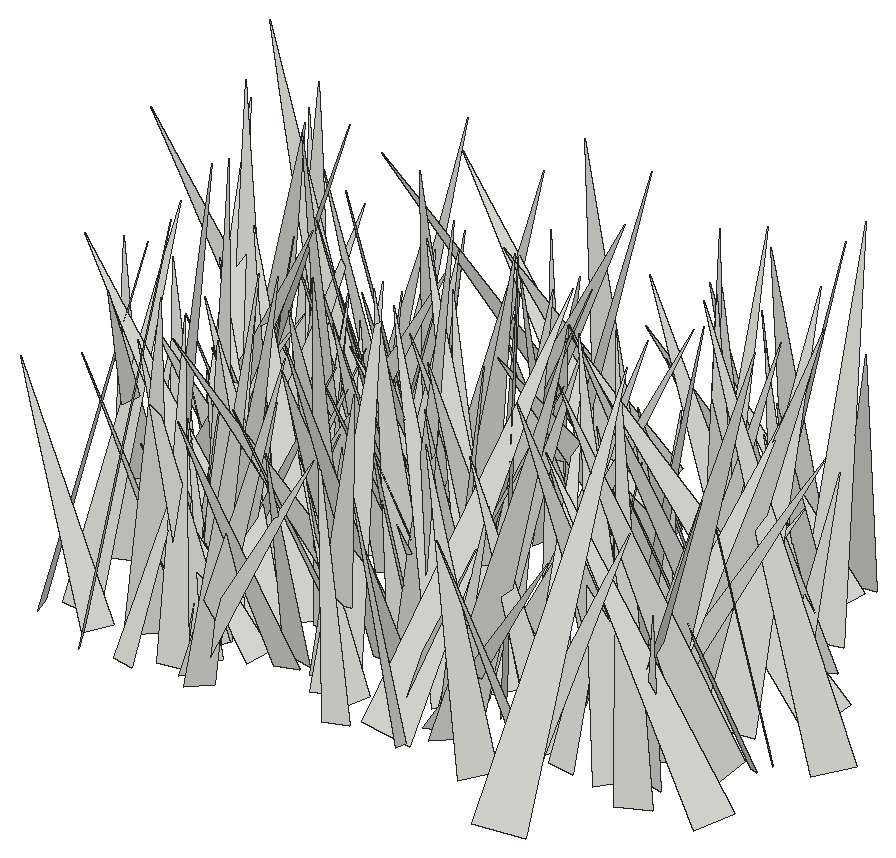
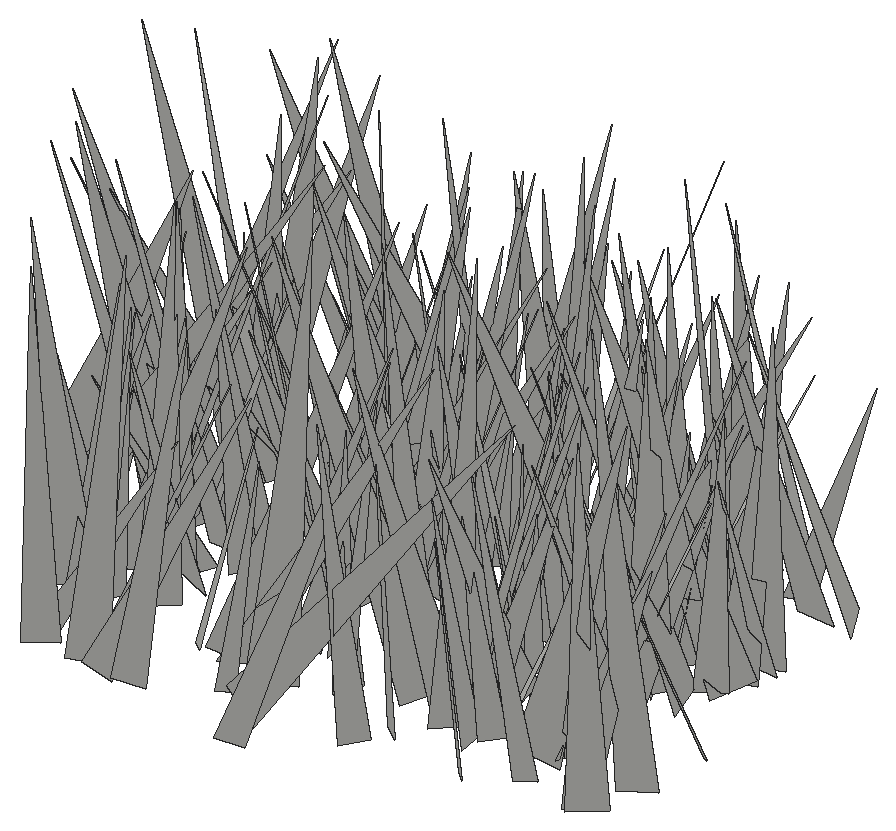
# SketchUp Ruby script. Lengths in inches.
U = 1.inch
M = Sketchup.active_model
def pt(a) = Geom::Point3d.new(a.map { |v| v * U })
def face(e, loops, mat)
  f = e.add_face(loops[0].map { |a| pt(a) })
  loops[1..].each { |l| e.add_face(l.map { |a| pt(a) }).erase! }
  f.material = f.back_material = mat if mat
  f
end
# faces: each face lists its corners as indices into pts; further lists are holes
def faces(e, pts, list, mat = nil) = list.each { |f| face(e, (f[0].is_a?(Array) ? f : [f]).map { |l| l.map { |i| pts[i] } }, mat) }
# xy, xz, yz: faces in a plane at the given z, y or x. An outline is a flat list of corners, or four numbers for a rectangle; further outlines are holes
def ring(l) = l.size == 4 ? [[l[0], l[1]], [l[2], l[1]], [l[2], l[3]], [l[0], l[3]]] : l.each_slice(2).to_a
def flat(e, list, mat, &to3) = list.each { |f| face(e, (f[0].is_a?(Array) ? f : [f]).map { |l| ring(l).map { |u, v| to3.(u, v) } }, mat) }
def xy(e, z, list, mat = nil) = flat(e, list, mat) { |x, y| [x, y, z] }
def xz(e, y, list, mat = nil) = flat(e, list, mat) { |x, z| [x, y, z] }
def yz(e, x, list, mat = nil) = flat(e, list, mat) { |y, z| [x, y, z] }
def lines(e, pts, list) = list.each { |a, b| e.add_line(pt(pts[a]), pt(pts[b])) }
# prism: a flat outline (further loops are holes) pulled along v
def prism(e, loops, v, mat = nil)
  f = face(e, loops, mat); d = Geom::Vector3d.new(v.map { |x| x * U })
  f.pushpull(f.normal.samedirection?(d) ? d.length : -d.length)
end
def box(e, o, s, mat = nil) = prism(e, [[o, [o[0] + s[0], o[1], o[2]], [o[0] + s[0], o[1] + s[1], o[2]], [o[0], o[1] + s[1], o[2]]]], [0, 0, s[2]], mat)
def at(x, y, z, deg = 0) = Geom::Transformation.translation(pt([x, y, z])) * Geom::Transformation.rotation(ORIGIN, Z_AXIS, deg.degrees)
def axes(o, x, y, z) = Geom::Transformation.new([*x, 0, *y, 0, *z, 0, *pt(o).to_a, 1])
def part(name) = M.definitions.add(name)
# library, detail: a bought-in or finely detailed component or shape, given as its bounding box
def library(name, o, s) = part(name).tap { |d| box(d.entities, o, s) }
def detail(e, o, s) = box(e.add_group.entities, o, s)
def put(e, d, t, mat = nil) = e.add_instance(d, t).tap { |i| i.material = mat if mat }
def group(e, t, mat = nil) = e.add_group.tap { |g| g.transformation = t; g.material = mat if mat }.entities
root = M.entities
c1 = part("fur_instance\#9")
p = [[0.8125,0,1.79],[0.67,-0.02,1.48],[0,-0.11,0],[0,0.11,0]]
faces(c1.entities,p,[[0,1,2,3]])
put(root,c1,axes([129.59,396.66,-27.1],[-4.54367,3.48057,1.82928],[3.81076,4.58683,0.73803],[0.96889,-1.71821,5.67579]))
put(root,c1,axes([114.01,396.57,-27.1],[-3.48001,3.233,0.8636],[3.33945,3.27515,1.19585],[-0.21495,-1.45934,4.59703]))
put(root,c1,axes([117.92,396.48,-27.1],[2.74788,4.31889,0.7575],[4.17328,-2.30167,-2.01583],[1.34551,-1.68135,4.70533]))
put(root,c1,axes([116.02,395.33,-27.1],[0.74131,3.87524,0.12897],[3.87698,-0.74271,0.03187],[-0.05555,-0.12068,3.94537]))
put(root,c1,axes([115.4,397.31,-27.1],[-4.12278,4.06528,3.37823],[4.64279,4.83304,-0.14992],[2.52655,-2.24755,5.78803]))
put(root,c1,axes([120.35,398.35,-27.1],[-0.32554,-5.06602,0.7464],[-4.99056,0.14633,-1.18345],[-1.14716,0.80105,4.9366]))
put(root,c1,axes([132.36,394.27,-27.1],[-3.86216,7.0455,1.20437],[6.7899,4.04407,-1.88376],[2.2331,-0.11104,7.81068]))
put(root,c1,axes([123.87,396.48,-27.1],[-0.78367,4.54033,1.31363],[4.69244,0.5877,0.76808],[-0.56674,-1.41222,4.54299]))
put(root,c1,axes([113.97,395.8,-27.1],[6.26441,4.08516,1.86388],[4.05019,-6.52197,0.68206],[-1.9387,-0.42509,7.44756]))
put(root,c1,axes([117.64,397.87,-27.1],[-4.95355,2.49117,1.9463],[2.93301,4.97148,1.10159],[1.17959,-1.90003,5.43416]))
put(root,c1,axes([130.23,398.35,-27.1],[-3.91317,-2.34388,0.53173],[-2.28614,3.94348,0.55853],[0.74167,-0.21123,4.52711]))
put(root,c1,axes([117.44,396.15,-27.1],[-0.20928,5.81187,1.2771],[5.90875,0.05179,0.73257],[-0.70395,-1.2931,5.76932]))
put(root,c1,axes([118.37,396.15,-27.1],[5.34451,-1.51745,2.02584],[-2.07356,-5.33917,1.4711],[-1.45157,2.03988,5.35746]))
put(root,c1,axes([131.07,396.62,-27.1],[0.51844,5.23573,1.343],[5.13497,-0.0558,-1.76472],[1.68777,-1.43851,4.95655]))
put(root,c1,axes([120.26,398.98,-27.1],[0.02895,-4.95019,0.58964],[-4.94989,0.0415,0.59139],[0.59214,0.58889,4.91483]))
put(root,c1,axes([126.4,396.66,-27.1],[-4.21104,-1.2398,0.43934],[-1.31531,3.95873,-1.43574],[-0.00925,1.50143,4.14832]))
put(root,c1,axes([125.05,397.93,-27.1],[3.85978,2.30102,0.3483],[2.28006,-3.60384,-1.45862],[0.46617,-1.42533,4.2503]))
put(root,c1,axes([117.06,397.82,-27.1],[-4.69197,-2.31538,0.05263],[-2.28134,4.60011,-1.00642],[-0.39908,0.92541,5.13447]))
put(root,c1,axes([121.87,398.7,-27.1],[3.13383,-5.16211,1.39491],[-5.34355,-3.08346,0.59403],[-0.19921,1.50298,6.00961]))
put(root,c1,axes([118.89,395.69,-27.1],[-6.51752,1.2418,2.00991],[0.54856,6.53189,-2.25684],[2.29801,1.9627,6.23913]))
put(root,c1,axes([119.2,398.35,-27.1],[-3.24563,2.42896,0.17461],[2.25293,2.88449,1.75171],[-0.92447,-1.49811,3.65588]))
put(root,c1,axes([122.88,400.67,-27.1],[-0.43608,-7.58063,0.50958],[-7.59761,0.43802,0.01424],[0.04352,0.50791,7.59315]))
put(root,c1,axes([118.24,397.18,-27.1],[-3.93894,0.78438,0.2139],[0.7314,3.88076,-0.76228],[0.35506,0.70765,3.94328]))
put(root,c1,axes([123.49,398.05,-27.1],[-4.0044,1.49429,0.5536],[1.5481,4.00291,0.3933],[0.37782,-0.56428,4.25599]))
put(root,c1,axes([122.49,398.78,-27.1],[-1.30736,-3.53096,1.01989],[-3.67333,1.2908,-0.2398],[0.12042,1.04076,3.75757]))
put(root,c1,axes([121.07,400.66,-27.1],[-3.83453,-4.44323,0.31037],[-4.29048,3.7947,1.3169],[1.19597,-0.63261,5.71941]))
put(root,c1,axes([126.65,398.21,-27.1],[3.7348,-2.45498,0.02516],[-2.33086,-3.53122,1.44009],[0.77113,1.21649,4.23106]))
put(root,c1,axes([117.09,397.07,-27.1],[2.12896,3.50938,0.78952],[3.35263,-2.26833,1.04217],[-1.30344,-0.10245,3.97015]))
put(root,c1,axes([127.47,398.07,-27.1],[7.2049,-3.47591,1.96261],[-3.83046,-7.15988,1.38131],[-1.1231,2.12096,7.87937]))
put(root,c1,axes([119.89,402.86,-27.1],[-6.50454,-4.83681,0.42708],[-4.2184,5.98256,3.50717],[2.40464,-2.5885,7.30777]))
put(root,c1,axes([111.64,396.65,-27.1],[5.51365,3.20537,1.24598],[2.89904,-5.59864,1.57419],[-1.84998,0.77981,6.18035]))
put(root,c1,axes([130.52,399.45,-27.1],[-4.35819,2.96505,1.59627],[3.3258,4.19926,1.28011],[0.52792,-1.97688,5.11338]))
put(root,c1,axes([133.25,400.75,-27.1],[1.43067,-7.01564,1.7352],[-6.90944,-1.84641,-1.76845],[-2.11892,1.28394,6.9382]))
put(root,c1,axes([137.39,399.07,-27.1],[-4.14935,5.21761,0.66717],[4.85978,3.47746,3.02911],[-2.01273,-2.35998,5.93844]))
put(root,c1,axes([120.62,402.08,-27.1],[5.40488,-4.57462,0.50738],[-4.27322,-5.27816,-2.06831],[-1.71004,-1.26929,6.77215]))
put(root,c1,axes([122.66,397.96,-27.1],[-3.77046,5.93467,2.17976],[6.06315,4.1134,-0.71146],[1.79161,-1.43096,6.99504]))
put(root,c1,axes([134.34,399.64,-27.1],[-0.14412,-3.47359,1.04669],[-3.58722,0.2928,0.47779],[0.54152,1.01518,3.44359]))
put(root,c1,axes([132.18,401.12,-27.1],[7.41722,0.99885,0.34739],[1.05742,-6.96886,-2.53978],[0.01548,-2.56338,7.04006]))
put(root,c1,axes([126.39,399.1,-27.1],[0.00091,-3.67707,1.93886],[-4.08733,0.35251,0.67045],[0.75747,1.90654,3.61543]))
put(root,c1,axes([112.81,397.18,-27.1],[0.72086,7.11073,0.81641],[7.15729,-0.71063,-0.13028],[0.04812,-0.82534,7.14599]))
put(root,c1,axes([133.4,399.15,-27.1],[-5.88987,4.84378,2.23578],[5.14185,6.04195,0.45575],[1.42207,-1.78441,7.61217]))
put(root,c1,axes([131.36,398.6875,-27.1],[0.22863,4.55848,1.01522],[4.65358,-0.13679,-0.43379],[0.39321,-1.03161,4.54355]))
put(root,c1,axes([135.82,401.57,-27.1],[-7.8024,0.71377,1.7229],[1.19599,7.6017,2.26696],[1.43089,-2.46171,7.49986]))
put(root,c1,axes([112.16,402.125,-27.1],[2.77965,-6.05851,0.20454],[-6.05263,-2.78627,-0.276],[-0.3362,0.0706,6.66001]))
put(root,c1,axes([118,400.26,-27.1],[-6.653,2.83628,0.09553],[2.75112,6.38619,1.99099],[-0.69638,-1.86767,6.95291]))
put(root,c1,axes([120.18,400.94,-27.1],[-0.4517,-7.27096,2.0225],[-7.50286,0.65147,0.6664],[0.81515,1.96726,7.25444]))
put(root,c1,axes([116.52,399.97,-27.1],[6.38697,-1.69717,1.73981],[-1.81592,-6.58358,0.24416],[-1.61547,0.69051,6.6041]))
put(root,c1,axes([125.53,396.96,-27.1],[-1.37451,8.097,0.63904],[7.82187,1.49419,-2.10823],[2.18815,-0.25501,7.93763]))
put(root,c1,axes([126.71,398.47,-27.1],[3.29752,4.92899,1.52703],[4.76096,-3.60504,1.35547],[-1.98997,-0.45731,5.77332]))
put(root,c1,axes([113.85,400.28,-27.1],[4.80804,6.17674,2.98381],[6.78482,-4.81897,-0.95722],[-1.01068,-2.96612,7.76873]))
put(root,c1,axes([134.84,398.1,-27.1],[-0.02832,7.80203,1.3013],[7.5934,-0.33756,2.1891],[-2.2148,-1.25708,7.48868]))
put(root,c1,axes([117.64,398.06,-27.1],[-7.86516,0.65945,1.92725],[0.13584,7.83978,-2.12819],[2.03241,2.02799,7.60042]))
put(root,c1,axes([116.55,400.14,-27.1],[3.89931,-1.45547,0.98195],[-1.58431,-3.9476,0.44006],[-0.75669,0.76505,4.13877]))
put(root,c1,axes([112.03,400.77,-27.1],[2.29625,-5.32789,2.30917],[-5.72704,-2.48806,-0.04565],[-0.95905,2.10109,5.80148]))
put(root,c1,axes([123.34,401.12,-27.1],[3.99451,-5.40043,2.70776],[-5.64329,-4.49426,-0.63847],[-2.15638,1.75774,6.68679]))
put(root,c1,axes([123.23,401.33,-27.1],[-1.72033,-4.15588,1.09836],[-4.2769,1.77348,0.01157],[0.4311,1.01028,4.49785]))
put(root,c1,axes([116.7,400.01,-27.1],[0.17252,3.92598,1.26935],[3.97591,-0.49782,0.99933],[-1.10305,-1.18034,3.80058]))
put(root,c1,axes([125.57,401.28,-27.1],[-2.41735,-5.08882,0.8159],[-4.81582,1.90935,-2.35956],[-1.83565,1.69223,5.11586]))
put(root,c1,axes([117.93,401.31,-27.1],[-5.02237,2.51021,1.68016],[2.86774,4.98644,1.12241],[0.94877,-1.78398,5.50142]))
put(root,c1,axes([125.96,399.85,-27.1],[-6.07575,2.79462,0.62219],[2.80321,6.10345,-0.04049],[0.58225,-0.22305,6.68752]))
put(root,c1,axes([123.87,400.02,-27.1],[3.41828,7.22194,2.57308],[7.56489,-3.63472,0.1519],[-1.24484,-2.25703,7.98861]))
put(root,c1,axes([115.95,400.16,-27.1],[-2.49427,4.27012,1.59064],[4.35584,2.76683,-0.59729],[1.33819,-1.04698,4.90903]))
put(root,c1,axes([118.85,399.21,-27.1],[-2.09774,5.99421,0.07606],[5.73274,1.98235,1.88224],[-1.75272,-0.69034,6.06533]))
put(root,c1,axes([116.13,399.85,-27.1],[4.9565,-0.0282,0.53243],[-0.1703,-4.80111,1.33099],[-0.50525,1.34155,4.77453]))
put(root,c1,axes([124.52,402.41,-27.1],[-3.87512,-3.17972,0.32504],[-3.163,3.88842,0.32938],[0.4601,-0.04943,5.00187]))
put(root,c1,axes([121.32,402.8,-27.1],[-2.38013,-2.88459,0.25848],[-2.75196,2.35686,0.96161],[0.90246,-0.42079,3.61403]))
put(root,c1,axes([125.82,403.23,-27.1],[3.87648,-5.20572,1.47803],[-5.00062,-4.14086,-1.46909],[-2.0683,0.2548,6.32205]))
put(root,c1,axes([127.39,400.72,-27.1],[6.18055,4.14964,3.19418],[4.26505,-6.85588,0.65402],[-3.03836,-1.18276,7.41558]))
put(root,c1,axes([125.02,402.26,-27.1],[-0.19276,-5.01478,1.27598],[-5.16585,0.1124,-0.33865],[-0.30027,1.28555,5.00705]))
put(root,c1,axes([118.4,403.67,-27.1],[4.15376,-5.21591,0.7578],[-5.12927,-4.22232,-0.94677],[-1.21268,-0.00681,6.60024]))
put(root,c1,axes([126.24,400.36,-27.1],[6.10707,-2.19869,2.10682],[-2.76305,-5.98564,1.76265],[-1.28003,2.43046,6.24689]))
put(root,c1,axes([123.23,403.76,-27.1],[-2.01035,-7.12989,1.00319],[-7.18316,2.0575,0.22838],[0.49393,0.90254,7.40437]))
put(root,c1,axes([132.33,401.64,-27.1],[6.94828,-4.27135,1.74082],[-4.55894,-6.83788,1.41876],[-0.70067,2.13364,8.03182]))
put(root,c1,axes([126.39,403.38,-27.1],[-6.42762,0.7775,0.36666],[0.8533,6.10569,2.01137],[0.10407,-2.04186,6.15412]))
put(root,c1,axes([118.98,401.12,-27.1],[-4.49285,4.90641,0.97236],[5.00159,4.41981,0.80831],[0.04935,-1.26349,6.60342]))
put(root,c1,axes([111.85,400.94,-27.1],[0.3484,4.1984,0.59349],[4.23915,-0.35779,0.04247],[-0.09183,-0.58788,4.21262]))
put(root,c1,axes([126.6,401.22,-27.1],[-5.45873,5.352,1.02249],[5.44819,5.38274,0.9113],[0.08123,-1.36725,7.5902]))
put(root,c1,axes([136.29,402.47,-27.1],[-3.48224,-3.77241,0.29956],[-3.58403,3.15695,-1.90663],[-1.21472,1.49981,4.76674]))
put(root,c1,axes([116.47,402.3125,-27.1],[3.59656,-0.31618,0.04156],[-0.31764,-3.59357,0.14939],[-0.02828,0.15246,3.60734]))
put(root,c1,axes([118.32,403.04,-27.1],[-3.2308,-2.41105,0.08917],[-2.40238,3.20101,-0.49122],[-0.22293,0.4467,4.00124]))
put(root,c1,axes([114.16,403.51,-27.1],[3.91302,0.34843,0.25725],[0.41449,-3.69091,-1.30566],[-0.12562,-1.32482,3.70519]))
put(root,c1,axes([111.92,402.53,-27.1],[6.68383,-3.60485,0.36068],[-3.59385,-6.50181,1.61538],[0.45749,1.59067,7.42019]))
put(root,c1,axes([130.04,402.55,-27.1],[-4.57594,-0.69447,0.70937],[-0.73517,4.61906,-0.2203],[0.6671,0.32667,4.62309]))
put(root,c1,axes([115.96,402.29,-27.1],[4.04604,3.23344,0.3968],[3.2461,-3.94826,-0.92578],[0.27467,-0.96906,5.09593]))
put(root,c1,axes([115.92,404.21,-27.1],[0.4513,-4.46287,0.47479],[-4.46772,-0.49211,-0.3789],[-0.42669,0.43236,4.4696]))
put(root,c1,axes([132.03,404.55,-27.1],[-2.1706,-3.79382,0.07549],[-3.76138,2.16267,0.53397],[0.50075,-0.20018,4.33814]))
put(root,c1,axes([113.86,403.37,-27.1],[2.36967,1.89121,2.13493],[2.35412,-2.86396,-0.07595],[-1.61018,-1.40392,3.03088]))
put(root,c1,axes([124.71,401.16,-27.1],[0.6459,3.9486,0.07217],[3.68247,-0.62859,1.43463],[-1.42692,0.16515,3.73504]))
put(root,c1,axes([136.28,403.38,-27.1],[-3.38614,-3.10021,1.02366],[-3.22386,3.40798,-0.34286],[0.51569,0.94841,4.57818]))
put(root,c1,axes([112.42,403.08,-27.1],[2.60909,-3.89298,2.22887],[-4.24925,-2.97119,-0.21539],[-1.4377,1.71676,4.68148]))
put(root,c1,axes([132.41,400.72,-27.1],[-1.13308,6.40977,0.66119],[6.08836,1.28481,-2.02171],[2.11049,-0.26515,6.18722]))
put(root,c1,axes([113.86,405.45,-27.1],[3.91388,-2.85851,1.41513],[-2.09693,-3.9939,-2.26798],[-2.40345,-1.17037,4.2832]))
put(root,c1,axes([118.05,402.07,-27.1],[0.83118,5.18677,1.07004],[5.28228,-0.88982,0.21009],[-0.38088,-1.02179,5.24874]))
put(root,c1,axes([129.16,402.85,-27.1],[-3.23487,-1.73884,2.61208],[-2.22596,3.91581,-0.14997],[2.2117,1.39779,3.66954]))
put(root,c1,axes([118.47,403.73,-27.1],[-2.90002,-7.26429,3.03178],[-7.85451,2.88308,-0.60516],[0.51793,3.0479,7.79832]))
put(root,c1,axes([115.9375,403.06,-27.1],[5.9864,-4.39629,0.74457],[-4.35138,-5.48795,2.58196],[0.97326,2.50473,6.96403]))
put(root,c1,axes([132.49,406.36,-27.1],[-7.22673,-3.69522,1.05519],[-3.3656,7.17065,2.06111],[1.85494,-1.38592,7.85061]))
put(root,c1,axes([122.51,403.11,-27.1],[4.96423,2.67259,0.04648],[2.6631,-4.93667,-0.5706],[0.22978,-0.52435,5.60898]))
put(root,c1,axes([131.36,403.31,-27.1],[4.19059,5.13354,0.34706],[4.85008,-3.79176,-2.47669],[1.71767,-1.81771,6.14657]))
put(root,c1,axes([119.16,405.38,-27.1],[1.67149,-5.33301,0.8085],[-5.34441,-1.75188,-0.5067],[-0.72935,0.6152,5.5658]))
put(root,c1,axes([115.84,404.49,-27.1],[-3.47734,-1.80435,0.22841],[-1.8088,3.48242,-0.02761],[0.19,0.12974,3.9175]))
put(root,c1,axes([124.07,403.47,-27.1],[-4.47005,3.93119,1.60818],[4.11701,4.5843,0.23722],[1.04438,-1.24571,5.94805]))
put(root,c1,axes([114.8,404.81,-27.1],[-3.58425,-2.16039,0.18109],[-2.16614,3.55434,-0.47063],[-0.08907,0.49634,4.15845]))
put(root,c1,axes([114.11,402.18,-27.1],[-5.29033,5.65073,1.03717],[5.57546,5.38985,-0.92613],[1.38587,-0.11308,7.68509]))
put(root,c1,axes([136.13,406.55,-27.1],[-7.44265,2.94787,0.75024],[2.95668,6.54484,3.6151],[-0.71474,-3.62229,7.14241]))
put(root,c1,axes([124.03,404.65,-27.1],[5.12868,-4.19399,1.94705],[-4.5125,-5.17419,0.74098],[-1.00889,1.82269,6.58361]))
put(root,c1,axes([125.23,404.25,-27.1],[5.08074,5.57509,0.64514],[5.46993,-4.72427,-2.25231],[1.25607,-1.97773,7.19879]))
put(root,c1,axes([115.9,405.44,-27.1],[-0.80392,-5.00028,1.94874],[-5.12712,1.2977,1.21465],[1.58527,1.66129,4.91668]))
put(root,c1,axes([131.92,404.11,-27.1],[6.06814,-4.77445,2.10475],[-5.2154,-5.64781,2.22478],[-0.15808,3.05854,7.39379]))
put(root,c1,axes([114.03,404.03,-27.1],[4.42151,2.80893,1.55928],[2.73673,-4.68252,0.67492],[-1.68278,-0.23477,5.19464]))
put(root,c1,axes([127.21,403.39,-27.1],[-2.44616,4.11048,0.29857],[4.09909,2.46258,-0.31948],[0.42742,-0.0923,4.7726]))
put(root,c1,axes([138.32,404.05,-27.1],[-2.68904,7.46116,1.26428],[7.06219,1.99214,3.26422],[-2.71897,-2.20471,7.22805]))
put(root,c1,axes([113.89,404.48,-27.1],[5.91163,-3.56463,4.13587],[-4.286,-6.80601,0.26026],[-3.38262,2.39395,6.89828]))
put(root,c1,axes([122.27,406.9,-27.1],[-5.24413,-0.63684,1.6828],[-0.10679,5.28634,1.66778],[1.7961,-1.54509,5.01248]))
put(root,c1,axes([129.49,404.6875,-27.1],[6.35559,1.23086,1.81432],[1.1106,-6.60444,0.5901],[-1.89033,0.25813,6.44673]))
put(root,c1,axes([112.67,404.08,-27.1],[7.43833,2.19546,1.23858],[2.06036,-7.51855,0.95355],[-1.45225,0.57818,7.69672]))
put(root,c1,axes([119.25,406.15,-27.1],[-2.70694,-4.99144,1.16007],[-5.08628,2.45713,-1.29614],[-0.62448,1.62351,5.52829]))
put(root,c1,axes([117.57,405.94,-27.1],[5.27684,1.71083,0.85913],[1.8324,-5.24307,-0.81398],[-0.55438,-1.04563,5.4872]))
put(root,c1,axes([134.07,403.95,-27.1],[-2.77927,7.20298,1.80131],[7.21654,3.07297,-1.15349],[1.74623,-1.2353,7.63392]))
put(root,c1,axes([118.89,406.6875,-27.1],[-4.07714,-4.72232,1.18622],[-4.85623,4.056,-0.54439],[0.3528,1.25658,6.21506]))
put(root,c1,axes([130.67,405.4375,-27.1],[2.74298,6.25055,1.8619],[6.47418,-2.36552,-1.59662],[0.78801,-2.32269,6.63657]))
put(root,c1,axes([117.35,406.84,-27.1],[-1.65671,-3.63214,1.3485],[-3.6613,1.94738,0.7471],[1.26719,0.87797,3.92161]))
put(root,c1,axes([129.11,406.23,-27.1],[-3.54773,2.23846,2.32232],[2.39169,4.14191,-0.33862],[2.16418,-0.90784,4.1812]))
put(root,c1,axes([126.16,410.9,-27.1],[6.60243,-3.6292,1.16999],[-2.40466,-5.77841,-4.35427],[-2.95933,-3.40161,6.14845]))
put(root,c1,axes([119.12,405.82,-27.1],[3.9195,-3.82723,2.46639],[-4.43668,-3.94163,0.93419],[-1.02305,2.43088,5.39791]))
put(root,c1,axes([120.66,407.62,-27.1],[0.32033,-6.88611,1.90206],[-6.92731,0.16595,1.76741],[1.74605,1.92169,6.66313]))
put(root,c1,axes([109.84,406.59,-27.1],[3.27011,3.05252,0.13659],[2.8317,-2.95233,-1.81533],[1.14804,-1.41282,4.08853]))
put(root,c1,axes([117.72,405.71,-27.1],[-2.46678,3.0111,0.36551],[3.02886,2.4705,0.08915],[0.1623,-0.33942,3.8915]))
put(root,c1,axes([118.68,407.39,-27.1],[-2.89225,-3.68575,0.79235],[-3.76683,2.78458,-0.79678],[-0.15371,1.11313,4.61682]))
put(root,c1,axes([113.37,409.17,-27.1],[-7.55604,-1.18176,1.01335],[-0.88861,7.39753,2.00103],[1.27821,-1.84315,7.38147]))
put(root,c1,axes([124.77,405.99,-27.1],[4.76351,-2.22786,1.63166],[-2.67424,-4.53288,1.61806],[-0.68857,2.19233,5.00362]))
put(root,c1,axes([132.32,405.27,-27.1],[-7.61718,0.0241,1.98426],[-0.51537,7.57673,-2.07045],[1.91631,2.1335,7.33043]))
put(root,c1,axes([121.25,406.3,-27.1],[6.06997,0.80019,0.53139],[0.73411,-6.05703,0.73529],[-0.61948,0.66277,6.07817]))
put(root,c1,axes([127.07,407.86,-27.1],[1.11597,-3.30458,1.27259],[-3.40234,-1.37051,-0.57526],[-0.98175,0.99326,3.44016]))
put(root,c1,axes([130.07,406.83,-27.1],[0.48143,3.7055,0.846],[3.27794,0.02687,-1.98307],[1.92393,-0.97302,3.16701]))
put(root,c1,axes([124.44,408.85,-27.1],[0.3349,-5.08877,0.86463],[-5.08924,-0.4702,-0.79617],[-0.86188,0.79915,5.03725]))
put(root,c1,axes([132.91,405.52,-27.1],[7.20277,3.49638,1.97973],[3.12762,-7.42996,1.74287],[-2.5223,0.77133,7.81454]))
put(root,c1,axes([130.77,407.77,-27.1],[4.6761,-4.10232,2.76945],[-4.45315,-5.14998,-0.1096],[-2.16064,1.73593,6.21956]))
put(root,c1,axes([117.37,406.46,-27.1],[1.88548,3.67223,0.79609],[3.49899,-2.04056,1.12569],[-1.36969,-0.15771,3.97154]))
put(root,c1,axes([117.53,410.09,-27.1],[7.0973,-2.99001,1.53723],[-2.6894,-7.20395,-1.59536],[-2.01752,-0.91535,7.53436]))
put(root,c1,axes([132.13,408.47,-27.1],[-5.92654,3.46188,1.28835],[3.68281,5.72588,1.55549],[0.28525,-1.99951,6.68498]))
put(root,c1,axes([134.06,408.92,-27.1],[0.22156,-4.52657,1.23949],[-4.53883,-0.5223,-1.09609],[-1.19379,1.1457,4.39744]))
put(root,c1,axes([110.2,409.62,-27.1],[1.15039,-7.47242,1.55869],[-7.41634,-0.72104,2.01691],[1.80677,1.79806,7.28646]))
put(root,c1,axes([116.54,408.06,-27.1],[-4.07706,-2.14403,0.24298],[-2.12817,3.90987,-1.20919],[-0.35608,1.18084,4.44491]))
put(root,c1,axes([112.15,407.39,-27.1],[0.82135,5.31818,1.14764],[5.3338,-0.55827,-1.23031],[1.07271,-1.29616,5.2387]))
put(root,c1,axes([111.73,410.52,-27.1],[1.96703,-4.29578,0.10046],[-4.18734,-1.94112,-1.01553],[-0.96439,-0.33368,4.61429]))
put(root,c1,axes([119.4,409.02,-27.1],[5.85705,-5.48153,0.51052],[-5.36351,-5.5136,2.33363],[1.24121,2.04104,7.67505]))
put(root,c1,axes([133.44,408.14,-27.1],[-1.54021,3.23682,1.39983],[3.28512,1.87235,-0.71486],[1.28237,-0.90889,3.51258]))
put(root,c1,axes([129.85,409.72,-27.1],[-4.92901,3.2655,3.81824],[4.17297,5.6397,0.56365],[2.798,-2.65855,5.88565]))
put(root,c1,axes([117.55,408.125,-27.1],[-2.16703,-5.16397,2.37315],[-5.48971,1.24499,-2.30381],[-1.47021,2.96275,5.10441]))
put(root,c1,axes([112.35,409.42,-27.1],[2.0816,-3.74764,1.04429],[-3.88491,-2.06538,0.3318],[-0.20701,1.076,4.27408]))
put(root,c1,axes([117.31,409.51,-27.1],[2.82941,3.82153,3.56935],[4.50896,-3.83832,0.53527],[-2.64833,-2.45217,4.72474]))
put(root,c1,axes([121.68,410.14,-27.1],[4.68677,-2.0034,0.66372],[-1.95488,-4.73014,-0.47351],[-0.79535,-0.17932,5.07496]))
put(root,c1,axes([133.05,409.41,-27.1],[0.28684,-3.45624,1.82339],[-3.70035,-0.82791,-0.9872],[-1.25608,1.64973,3.32465]))
put(root,c1,axes([121.99,409.77,-27.1],[6.05057,5.41917,1.99571],[5.77348,-5.74186,-1.9125],[-0.1309,-2.76104,7.89425]))
put(root,c1,axes([131.96,411.17,-27.1],[4.64418,-2.47093,1.08294],[-2.19439,-4.71399,-1.3452],[-1.56935,-0.72073,5.0857]))
put(root,c1,axes([127.18,411.03,-27.1],[-2.4025,-2.92839,0.44923],[-2.80853,2.4353,0.85486],[0.94311,-0.20767,3.69008]))
put(root,c1,axes([123.61,408.13,-27.1],[-5.70107,0.73605,0.76728],[0.48907,5.53142,-1.67238],[0.94409,1.57933,5.49974]))
put(root,c1,axes([121.36,410.86,-27.1],[-1.65824,-4.82946,1.36253],[-4.95542,1.80194,0.35604],[0.78993,1.16588,5.09379]))
put(root,c1,axes([131.42,410.3,-27.1],[-4.23654,2.45749,2.21286],[2.8358,4.54981,0.37637],[1.70124,-1.46429,4.88322]))
put(root,c1,axes([118.69,408.77,-27.1],[6.30569,-0.68619,2.05979],[-1.17683,-6.39727,1.4715],[-1.82446,1.75482,6.16987]))
put(root,c1,axes([121.23,410.75,-27.1],[-1.26744,-3.38882,1.28492],[-3.35573,1.6115,0.94004],[1.36901,0.81271,3.49382]))
put(root,c1,axes([130.38,411.27,-27.1],[-4.86082,-0.82699,0.28427],[-0.77768,4.82218,0.73078],[0.39992,-0.67448,4.87621]))
put(root,c1,axes([116.79,407.24,-27.1],[-6.46453,1.71895,1.7422],[0.79023,6.12289,-3.109],[2.31637,2.70842,5.92275]))
put(root,c1,axes([131.86,410.125,-27.1],[-3.13424,-4.33981,2.11732],[-4.81159,3.01955,-0.93345],[0.40688,2.2779,5.27125]))
put(root,c1,axes([115.95,409.88,-27.1],[2.7326,-2.75522,2.01665],[-3.2693,-2.85632,0.52755],[-0.98478,1.83723,3.84448]))
put(root,c1,axes([123.83,411.41,-27.1],[3.74176,-6.61768,2.63887],[-6.89022,-4.11933,-0.5604],[-1.81167,1.99888,7.58159]))
put(root,c1,axes([114.12,409.95,-27.1],[-2.60972,7.0339,1.93347],[7.14895,2.0575,2.16424],[-1.45142,-2.51309,7.18348]))
put(root,c1,axes([125.45,411.02,-27.1],[-6.72983,3.60579,0.05795],[3.45053,6.40273,2.3226],[-1.04828,-2.07339,7.27309]))
put(root,c1,axes([111.04,411.79,-27.1],[2.15592,-3.18911,0.31319],[-3.19535,-2.16794,-0.07942],[-0.24138,0.21478,3.84865]))
put(root,c1,axes([113.45,411.35,-27.1],[0.14432,-5.01914,1.5992],[-4.96199,0.40759,1.72702],[1.76858,1.55311,4.71487]))
put(root,c1,axes([130.01,407.84,-27.1],[1.21236,6.8418,0.01969],[6.58716,-1.17263,1.87473],[-1.84929,0.30844,6.6907]))
put(root,c1,axes([116.36,410.47,-27.1],[4.45017,0.43948,1.54669],[0.28501,-4.6951,0.51402],[-1.58245,0.39027,4.44218]))
put(root,c1,axes([112.84,409.47,-27.1],[-0.8171,5.77252,0.59098],[5.63961,0.64951,1.4532],[-1.36602,-0.77139,5.64605]))
put(root,c1,axes([124.64,412.77,-27.1],[3.47774,-1.50181,0.39234],[-1.2719,-3.30895,-1.39185],[-0.88975,-1.13996,3.5232]))
put(root,c1,axes([110.64,411.64,-27.1],[3.75494,-4.9741,2.2471],[-5.32599,-3.93562,0.18806],[-1.1937,1.91308,6.22943]))
put(root,c1,axes([118.77,411.58,-27.1],[2.85129,3.39796,1.84964],[3.79237,-2.9092,-0.50161],[-0.76499,-1.75715,4.40731]))
put(root,c1,axes([132.7,410.36,-27.1],[-2.30774,6.81626,2.09214],[7.04491,2.51871,-0.43516],[1.09893,-1.8327,7.18315]))
put(root,c1,axes([123.64,413.25,-27.1],[-2.19661,-7.3796,0.4517],[-6.30745,1.62463,-4.13089],[-3.85727,1.54587,6.49764]))
put(root,c1,axes([122.45,415.3125,-27.1],[6.08199,-2.63161,2.26399],[-1.13407,-5.82276,-3.72169],[-3.281,-2.8656,5.48316]))
put(root,c1,axes([119.32,412.8,-27.1],[4.77577,-2.2799,0.31782],[-2.26651,-4.78515,-0.26858],[-0.40236,-0.10607,5.28524]))
put(root,c1,axes([115.26,412.41,-27.1],[2.93725,2.51058,1.33666],[2.80043,-2.8887,-0.72813],[-0.49727,-1.43859,3.79478]))
put(root,c1,axes([131.31,413.97,-27.1],[2.32461,-5.72045,0.33614],[-5.68592,-2.25756,0.90225],[0.71192,0.64824,6.10846]))
put(root,c1,axes([128.68,414.34,-27.1],[0.56796,-5.36738,0.34113],[-5.01782,-0.65229,-1.90884],[-1.93561,0.11605,5.04853]))
put(root,c1,axes([131.78,413.1,-27.1],[-4.01783,2.35497,0.3103],[2.27352,3.63609,1.84258],[-0.68795,-1.73727,4.27712]))
put(root,c1,axes([129.34,414.02,-27.1],[2.40943,-6.40182,1.38295],[-6.51779,-2.4885,-0.16399],[-0.64358,1.23501,6.83826]))
put(root,c1,axes([127.42,414.31,-27.1],[0.8568,-5.86099,0.80486],[-5.91149,-0.87995,-0.11477],[-0.231,0.77949,5.92218]))
